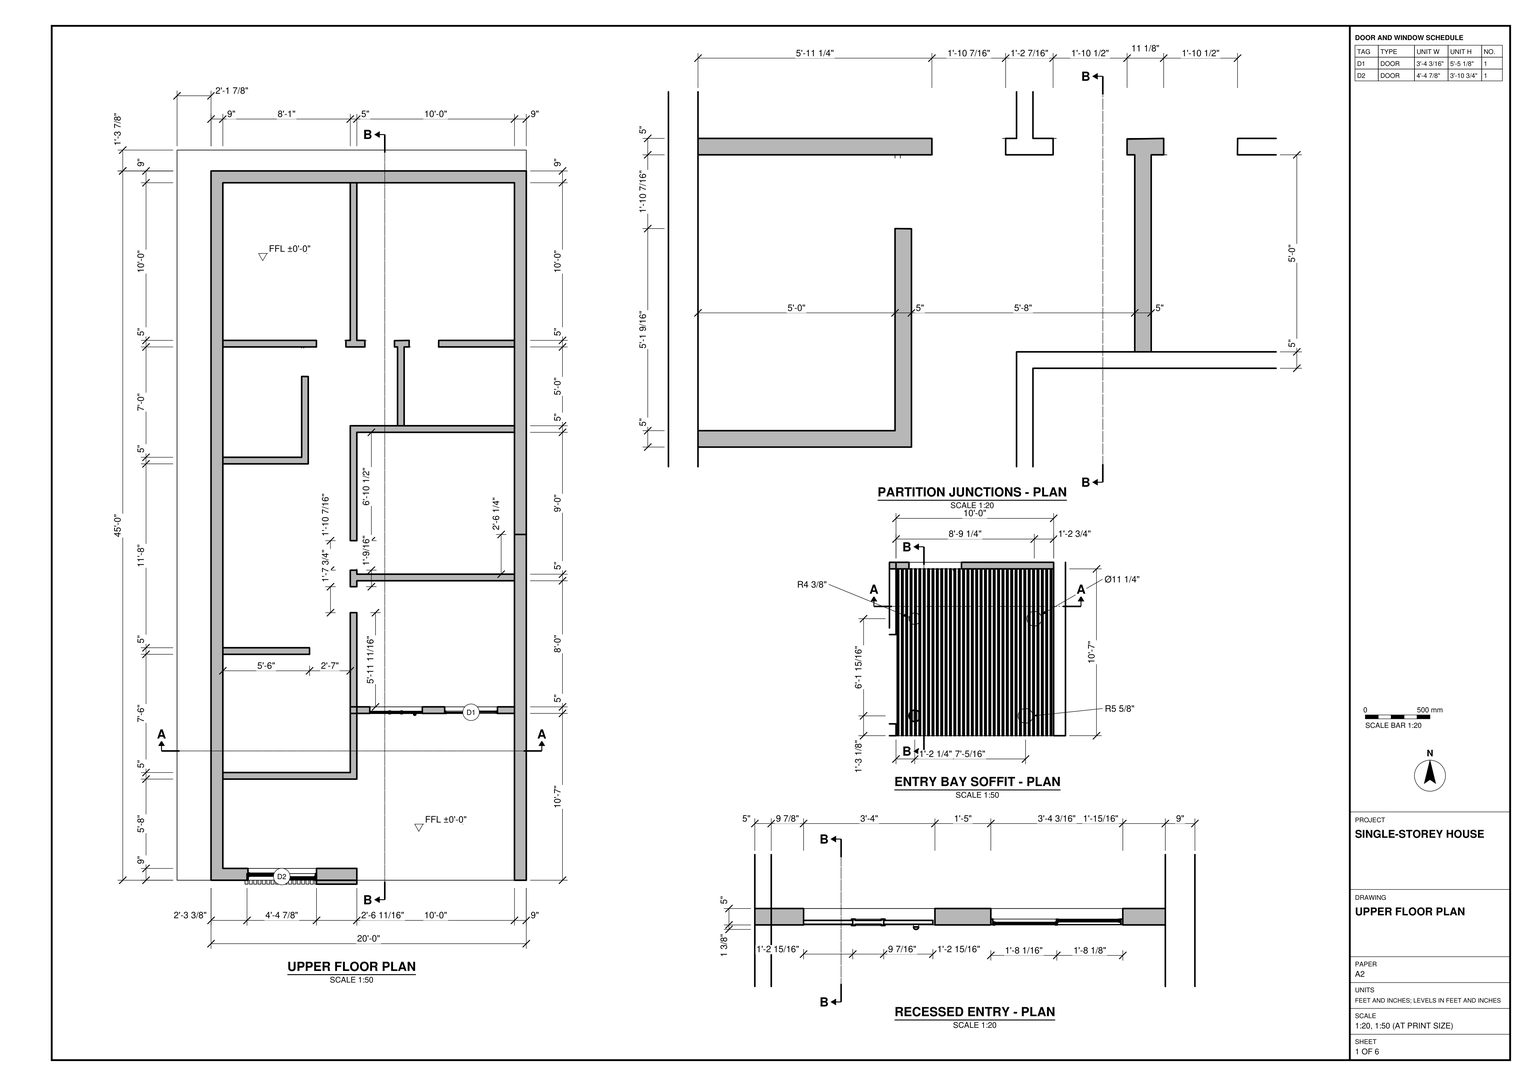
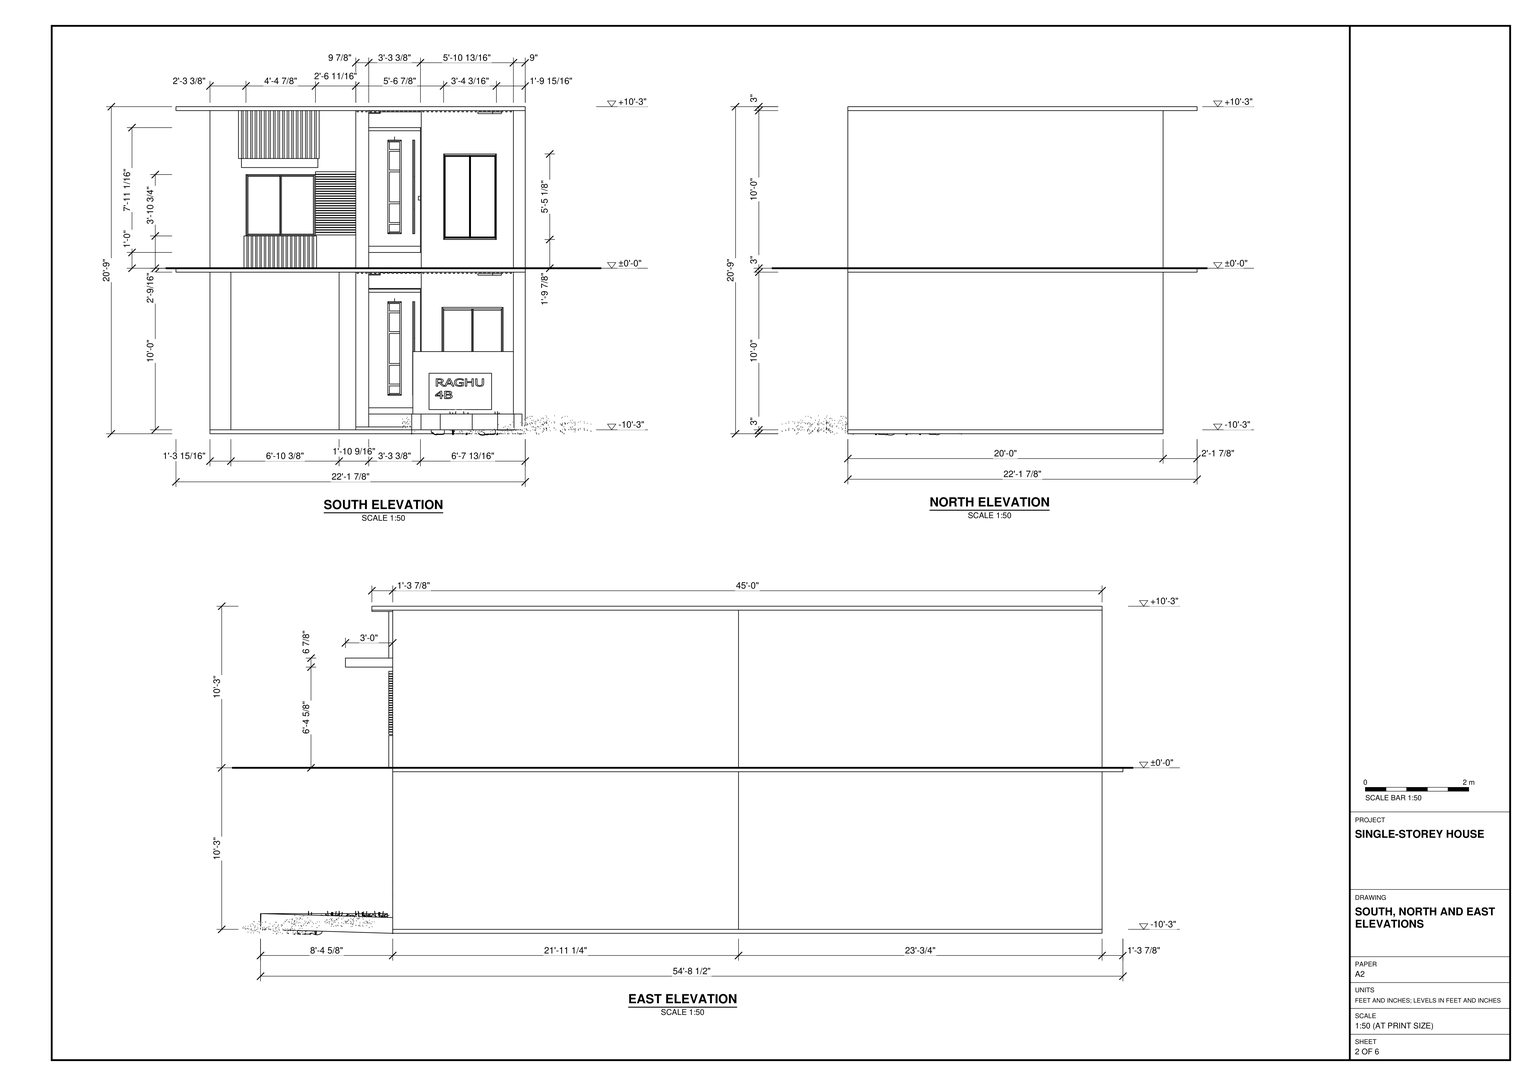
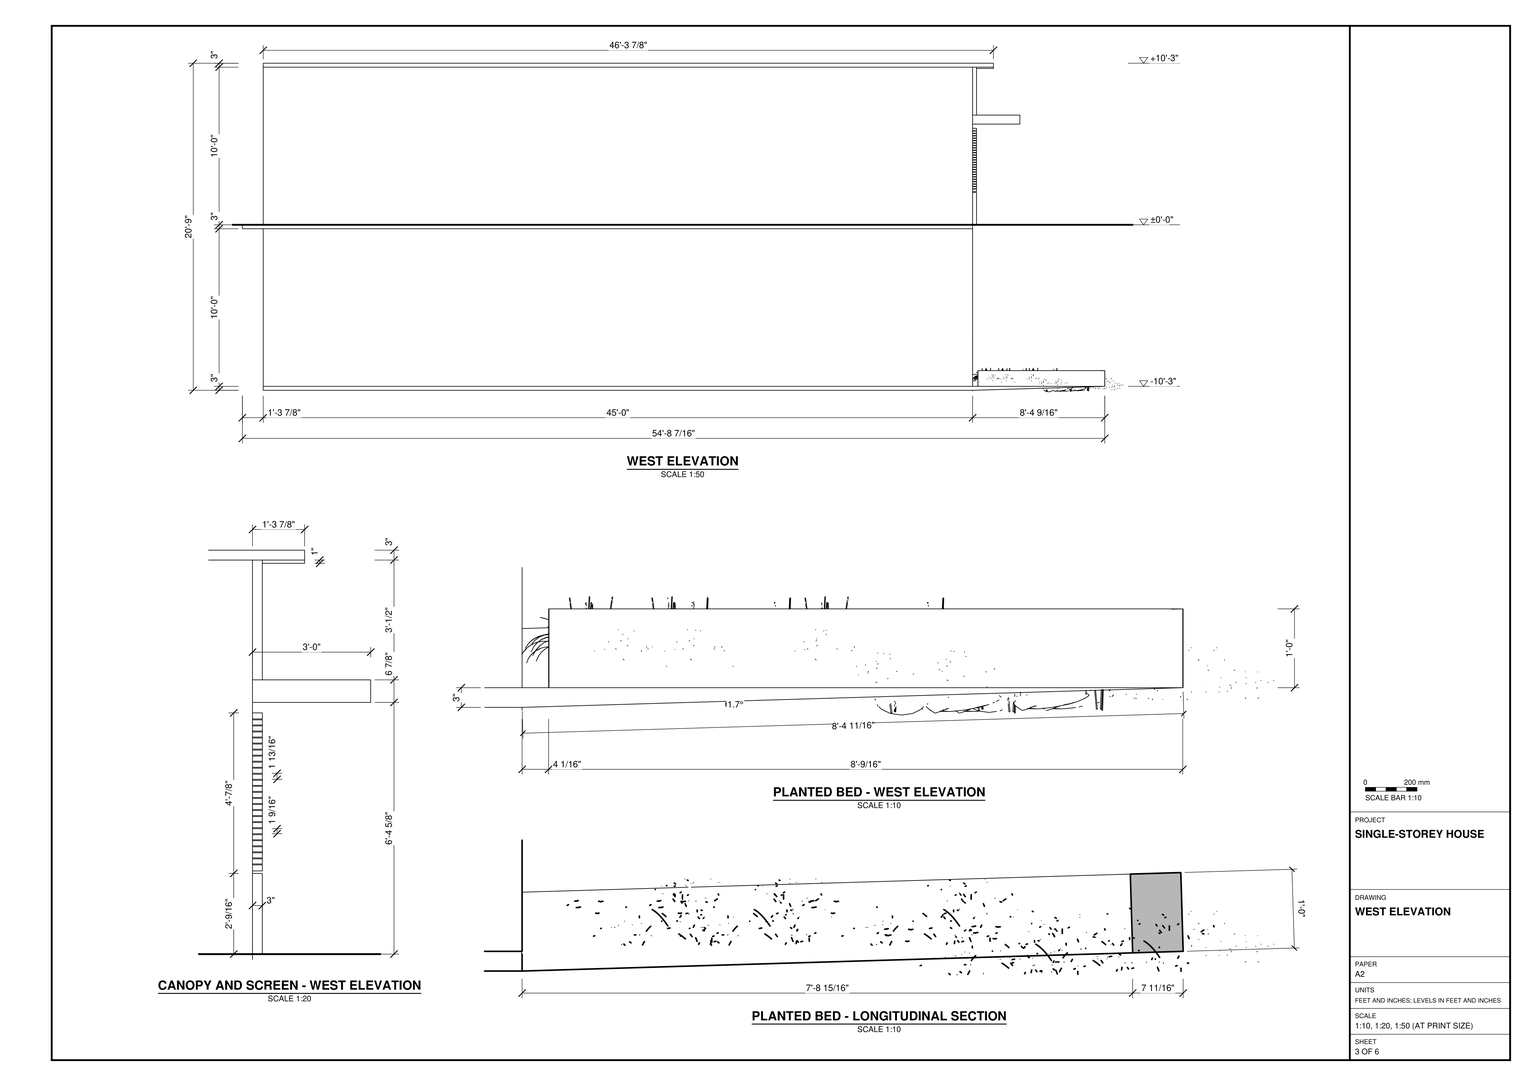
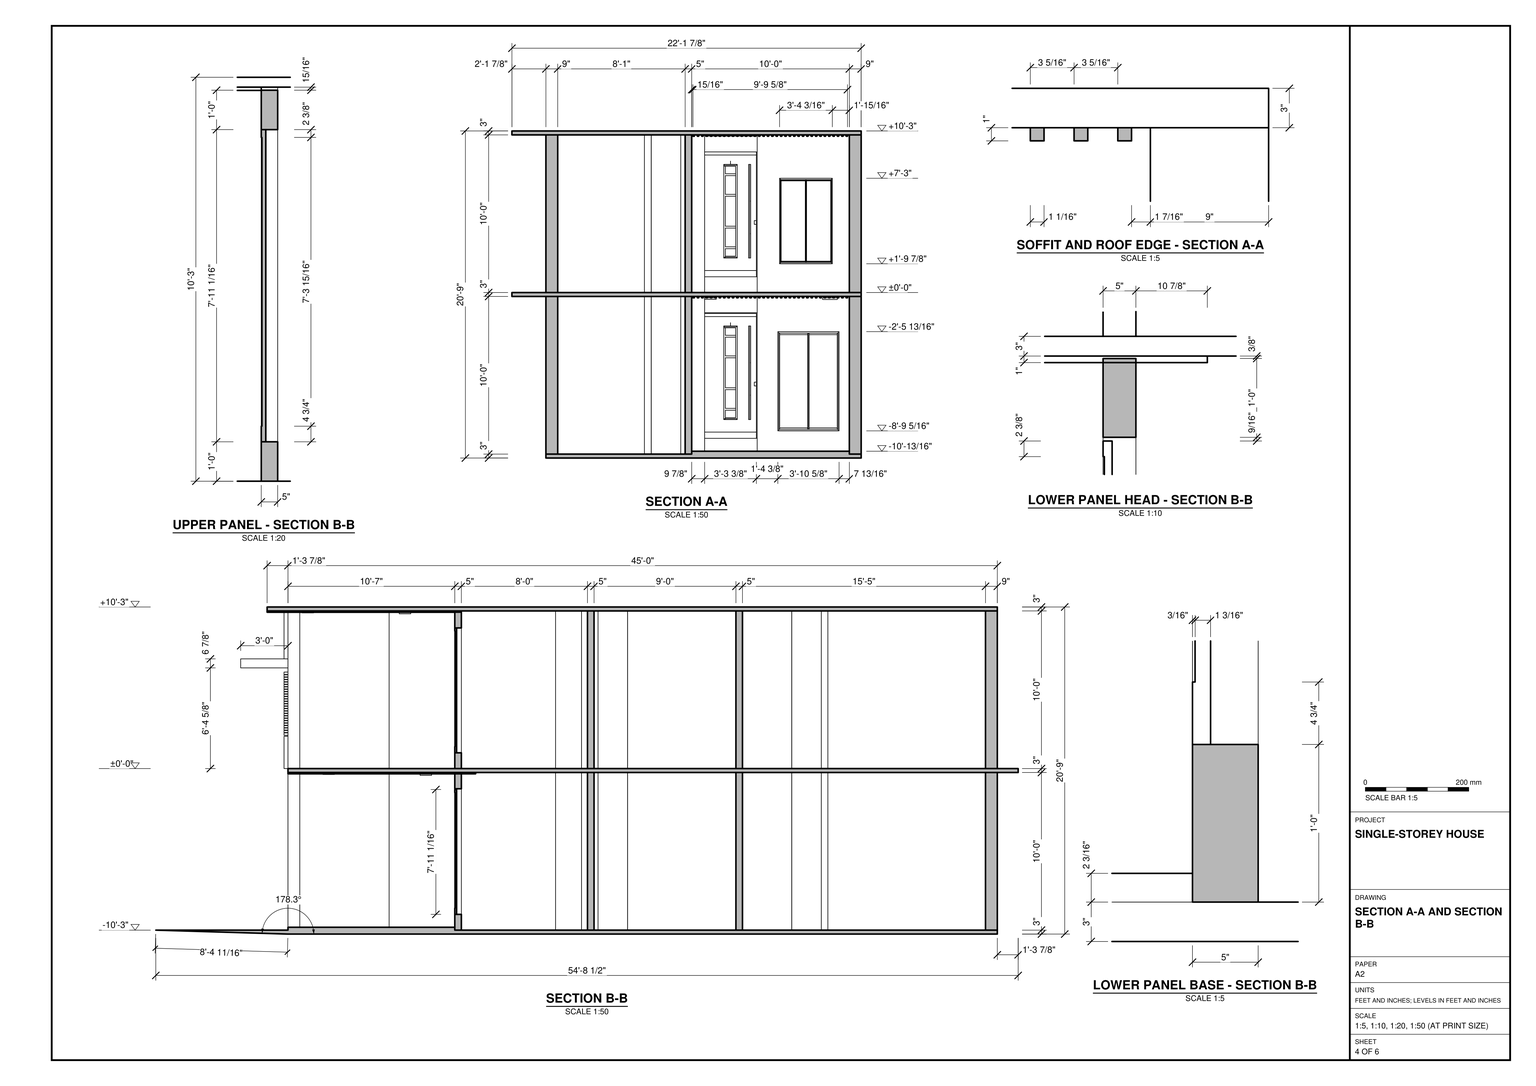
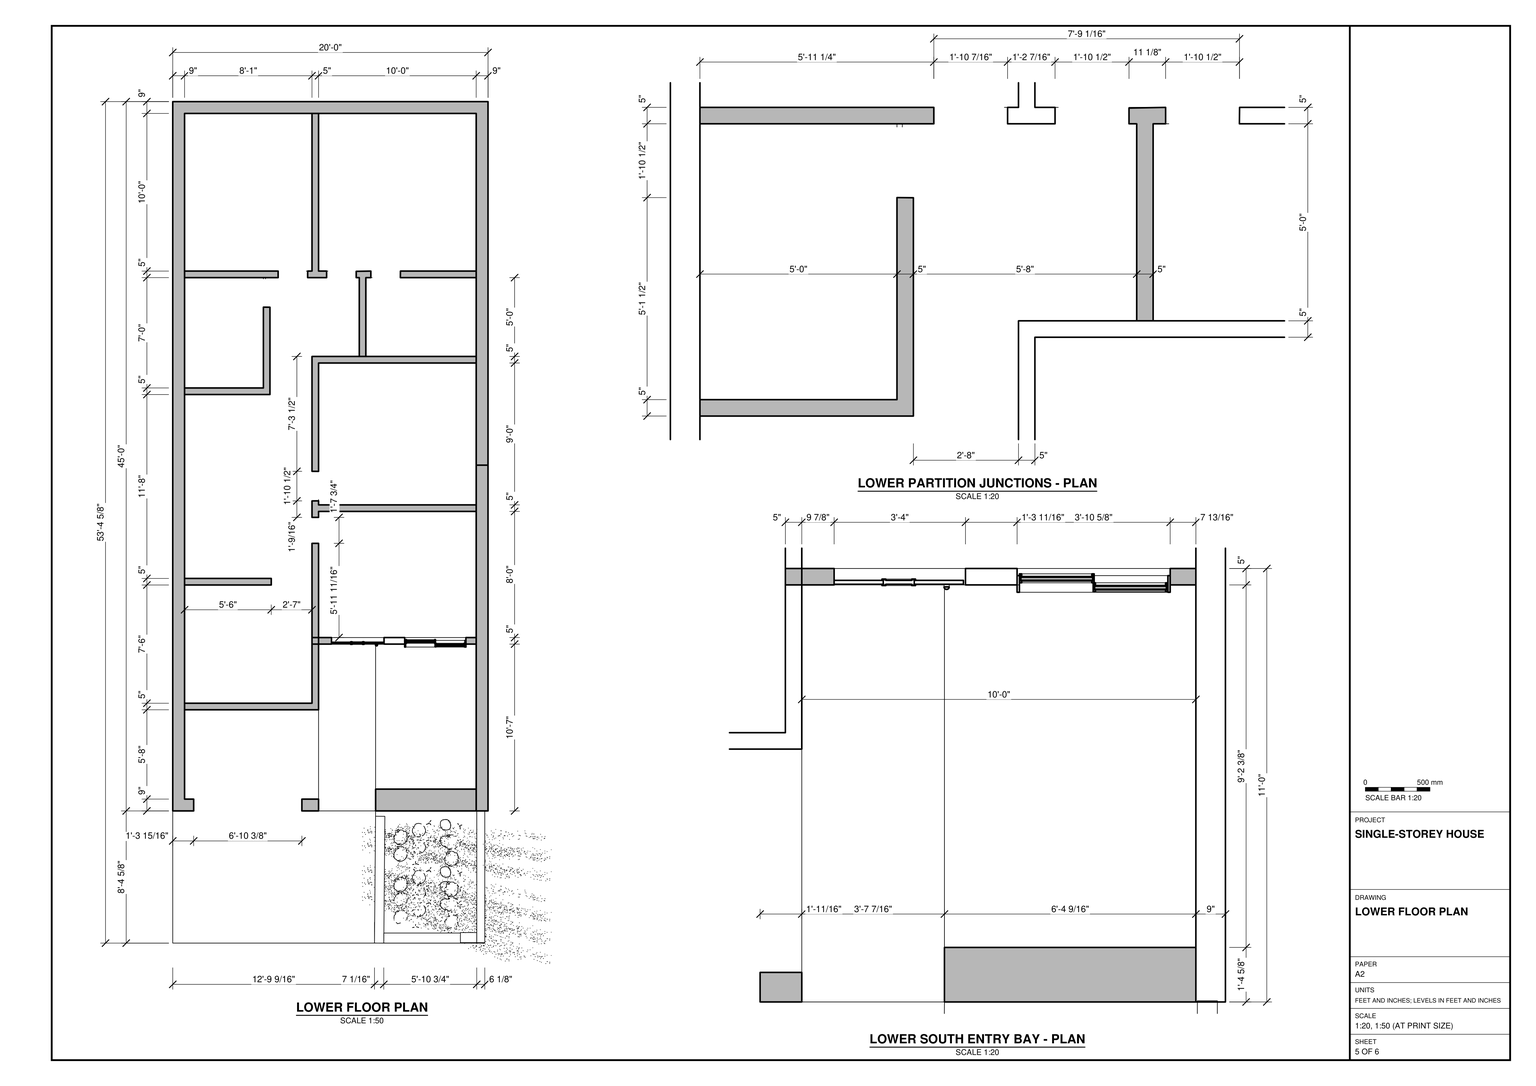
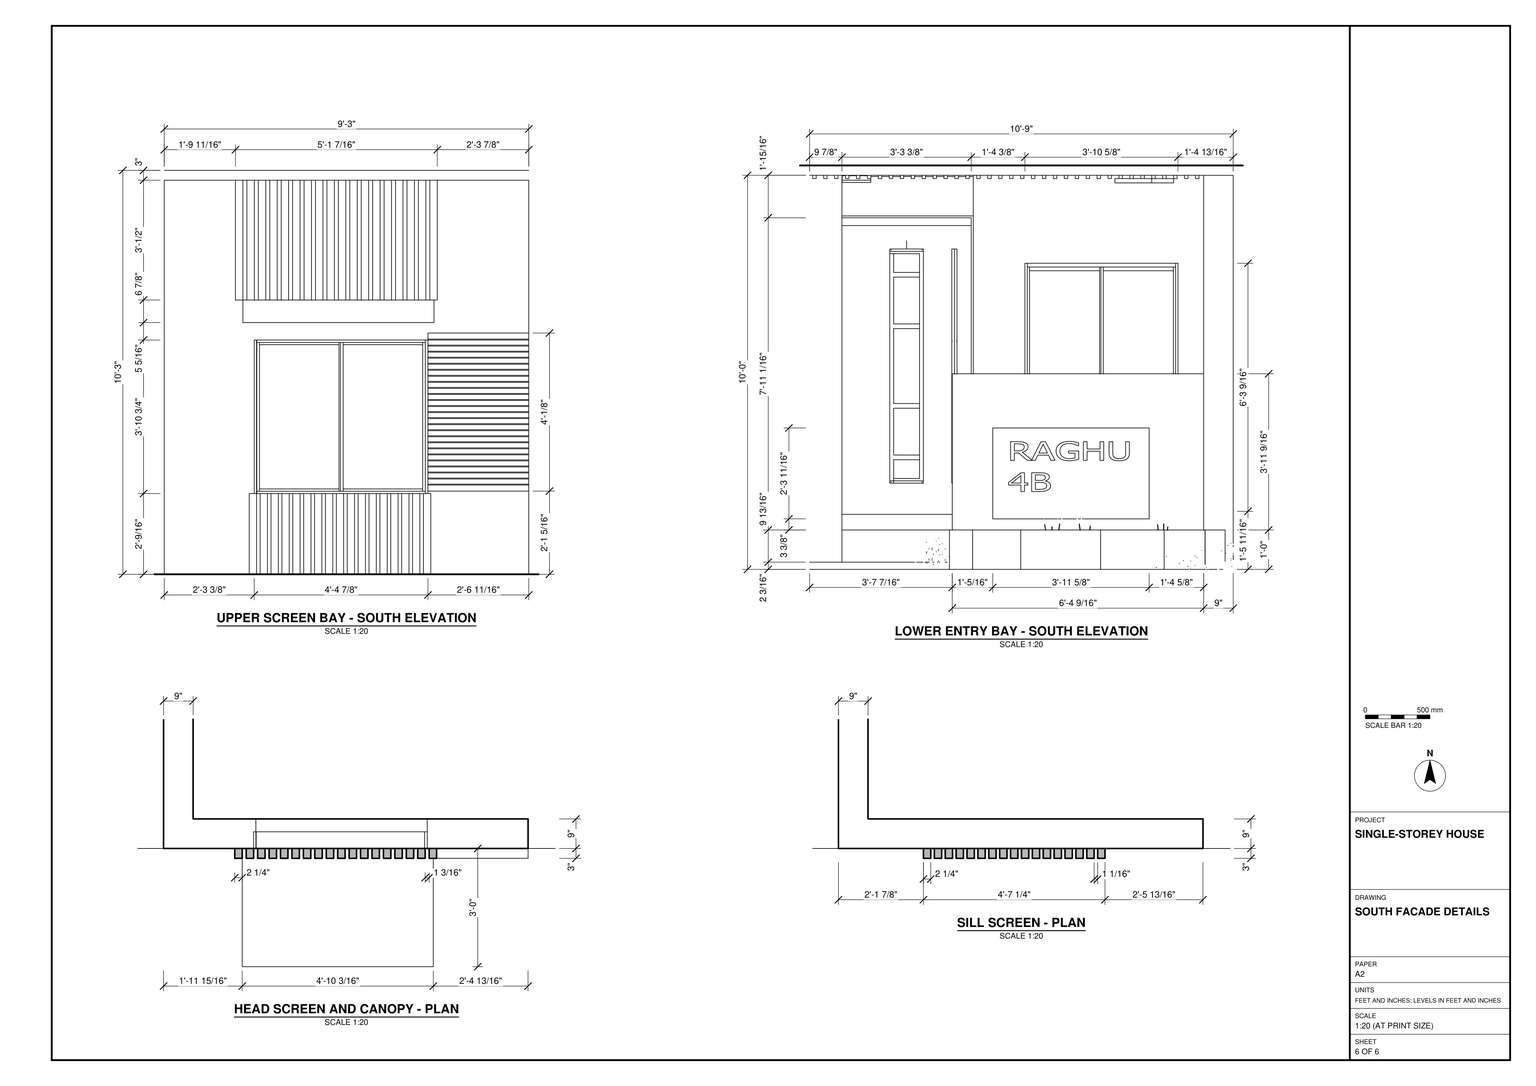
Build the house in SketchUp from task_files/diagram_01.pdf. Work in feet and inches. Use the finished floor of the partitioned plan as the ±0'-0" datum. The complete model, including projections and planting, measures 26'-4 5/16" across (x), 56'-2 5/16" front to back (y) and 20'-10 13/16" high (z).

Lay out the 20'-0" by 45'-0" house footprint with 9" exterior walls. Follow the plan and enlarged junction detail for the 5" partitions, including their short returns and the gaps between rooms. Use the elevations to build the enclosure below the datum floor as well as the walls above it. Match the thin slab edges and overhangs at the floor and flat roof; keep the side and rear walls plain as drawn.

On the south front, set the entrance back from the outer wall line. Model the framed openings, scheduled door units, slatted entry soffit, projecting canopy and screen. Use the south elevation to align the upper and lower entrance panels. Extend the low planted bed in front of the lower façade as shown in the west elevation and section. Decor and loose items, including plants, may be any suitable library components.

Keep walls, slabs, roof and each furniture or joinery piece shown in separate groups or components, and use components for repeated parts. Save one SketchUp model as output_files/house_with_its_recessed_entrance_and_planted_bed.skp.

# SketchUp Ruby script. Lengths in inches.
U = 1.inch
M = Sketchup.active_model
def pt(a) = Geom::Point3d.new(a.map { |v| v * U })
def face(e, loops, mat)
  f = e.add_face(loops[0].map { |a| pt(a) })
  loops[1..].each { |l| e.add_face(l.map { |a| pt(a) }).erase! }
  f.material = f.back_material = mat if mat
  f
end
# faces: each face lists its corners as indices into pts; further lists are holes
def faces(e, pts, list, mat = nil) = list.each { |f| face(e, (f[0].is_a?(Array) ? f : [f]).map { |l| l.map { |i| pts[i] } }, mat) }
# xy, xz, yz: faces in a plane at the given z, y or x. An outline is a flat list of corners, or four numbers for a rectangle; further outlines are holes
def ring(l) = l.size == 4 ? [[l[0], l[1]], [l[2], l[1]], [l[2], l[3]], [l[0], l[3]]] : l.each_slice(2).to_a
def flat(e, list, mat, &to3) = list.each { |f| face(e, (f[0].is_a?(Array) ? f : [f]).map { |l| ring(l).map { |u, v| to3.(u, v) } }, mat) }
def xy(e, z, list, mat = nil) = flat(e, list, mat) { |x, y| [x, y, z] }
def xz(e, y, list, mat = nil) = flat(e, list, mat) { |x, z| [x, y, z] }
def yz(e, x, list, mat = nil) = flat(e, list, mat) { |y, z| [x, y, z] }
def lines(e, pts, list) = list.each { |a, b| e.add_line(pt(pts[a]), pt(pts[b])) }
# prism: a flat outline (further loops are holes) pulled along v
def prism(e, loops, v, mat = nil)
  f = face(e, loops, mat); d = Geom::Vector3d.new(v.map { |x| x * U })
  f.pushpull(f.normal.samedirection?(d) ? d.length : -d.length)
end
def box(e, o, s, mat = nil) = prism(e, [[o, [o[0] + s[0], o[1], o[2]], [o[0] + s[0], o[1] + s[1], o[2]], [o[0], o[1] + s[1], o[2]]]], [0, 0, s[2]], mat)
def at(x, y, z, deg = 0) = Geom::Transformation.translation(pt([x, y, z])) * Geom::Transformation.rotation(ORIGIN, Z_AXIS, deg.degrees)
def axes(o, x, y, z) = Geom::Transformation.new([*x, 0, *y, 0, *z, 0, *pt(o).to_a, 1])
def part(name) = M.definitions.add(name)
# library, detail: a bought-in or finely detailed component or shape, given as its bounding box
def library(name, o, s) = part(name).tap { |d| box(d.entities, o, s) }
def detail(e, o, s) = box(e.add_group.entities, o, s)
def put(e, d, t, mat = nil) = e.add_instance(d, t).tap { |i| i.material = mat if mat }
def group(e, t, mat = nil) = e.add_group.tap { |g| g.transformation = t; g.material = mat if mat }.entities
root = M.entities
M.materials.add("Emissive\#1").color = [255, 185, 108]
M.materials.add("Glass_Tinted_Gray").color = [0, 0, 0]
M.materials["Glass_Tinted_Gray"].alpha = 0.125
M.materials.add("[0135_DarkGray]").color = [81, 81, 81]
M.materials.add("[Field Rectangle Tile]").color = [196, 189, 179]
M.materials.add("[Granite Dark Gray]").color = [69, 68, 68]
M.materials.add("[Marble Carrara Gold Floor Tile]").color = [225, 223, 217]
M.materials.add("[Mirror 02]").color = [229, 229, 229]
M.materials.add("[Terrazzo Light Blue]").color = [196, 214, 227]
M.materials.add("[Tile Navy]").color = [43, 47, 58]
M.materials.add("[Wood Bamboo]").color = [177, 105, 43]
M.materials.add("[Wood Veneer 01]").color = [120, 70, 37]
c1 = part("PENTEK_RP Fineline 50S_Sliding_DoorCase_E1")
box(c1.entities,[0,0,0],[1.51,3.66,99.27],"[0135_DarkGray]")
c2 = part("PENTEK_RP Fineline 50S_SlidingDooe_Case_E2")
box(c2.entities,[0,0,0],[96.25,3.66,1.51],"[0135_DarkGray]")
c3 = part("pentek_RP Fineline 50S_SlidingDoor_Case")
put(c3.entities,c1,at(97.76,0,0))
put(c3.entities,c2,at(1.51,0,0))
put(c3.entities,c1,at(0,0,0))
put(c3.entities,c2,at(1.51,0,97.76))
c4 = part("PENTEK_RP Fineline 50S_SlidingDoor_GlazingBead_2")
box(c4.entities,[0,0,0],[0.56,0.59,94.39],"[0135_DarkGray]")
c5 = part("PENTEK_RP Fineline 50S_SlidingDoor_Glass")
box(c5.entities,[0,0,0],[46.58,0.16,94.39],"Glass_Tinted_Gray")
c6 = part("PENTEK_RP Fineline 50S_SlidingDoor_GlazingBead")
box(c6.entities,[0,0,0],[45.47,0.59,0.56],"[0135_DarkGray]")
c7 = part("PENTEK_RP Fineline 50S_SlidingDoor_Leaf_E1")
xy(c7.entities,0,[[0,0,0.93,1.97],[0.93,1.57,1.49,1.97]],"[0135_DarkGray]")
xy(c7.entities,96.25,[[0,0,0.93,0,0.93,1.57,1.49,1.57,1.49,1.97,0,1.97]],"[0135_DarkGray]")
xz(c7.entities,0,[[0,0,0.93,96.25]],"[0135_DarkGray]")
xz(c7.entities,1.57,[[0.93,0,1.49,95.32],[0.93,95.32,1.49,96.25]],"[0135_DarkGray]")
xz(c7.entities,1.97,[[0,0,1.49,96.25]],"[0135_DarkGray]")
yz(c7.entities,0,[[0,0,1.97,96.25]],"[0135_DarkGray]")
yz(c7.entities,0.93,[[0,0,1.57,0.93],[0,0.93,1.57,95.32],[0,95.32,1.57,96.25]],"[0135_DarkGray]")
yz(c7.entities,1.49,[[1.57,0,1.97,95.32],[1.57,95.32,1.97,96.25]],"[0135_DarkGray]")
c8 = part("PENTEK_RP Fineline 50S_SlidingDoor_Leaf_E2")
xy(c8.entities,0,[[0,0,0,1.57,0.56,1.57,0.56,1.97,46.02,1.97,46.02,1.57,46.58,1.57,46.58,0]],"[0135_DarkGray]")
xy(c8.entities,0.93,[[0,0,46.58,1.57]],"[0135_DarkGray]")
xy(c8.entities,1.49,[[0.56,1.57,46.02,1.97]],"[0135_DarkGray]")
xz(c8.entities,0,[[0,0,46.58,0.93]],"[0135_DarkGray]")
xz(c8.entities,1.57,[[0,0,0.56,0.93],[46.02,0,46.58,0.93],[0.56,0.93,46.02,1.49]],"[0135_DarkGray]")
xz(c8.entities,1.97,[[0.56,0,46.02,1.49]],"[0135_DarkGray]")
yz(c8.entities,0,[[0,0,1.57,0.93]],"[0135_DarkGray]")
yz(c8.entities,0.56,[[1.57,0,1.97,0.93],[1.57,0.93,1.97,1.49]],"[0135_DarkGray]")
yz(c8.entities,46.02,[[1.57,0,1.97,0.93],[1.57,0.93,1.97,1.49]],"[0135_DarkGray]")
yz(c8.entities,46.58,[[0,0,1.57,0.93]],"[0135_DarkGray]")
c9 = part("PENTEK_RP Fineline S_SlidingDoor_Leaf1")
put(c9.entities,c4,at(0.93,0,0.93))
put(c9.entities,c4,at(46.96,0,0.93))
put(c9.entities,c5,at(1.49,1.42,0.93))
put(c9.entities,c6,at(1.49,0,0.93))
put(c9.entities,c5,at(1.49,0.59,0.93),"[Terrazzo Light Blue]")
put(c9.entities,c7,at(0,0,0))
put(c9.entities,c7,axes([48.44,0,0],[-1,0,0],[0,1,0],[0,0,1]))
put(c9.entities,c8,axes([0.93,0,96.25],[1,0,0],[0,1,0],[0,0,-1]))
put(c9.entities,c8,at(0.93,0,0))
put(c9.entities,c6,at(1.49,0,94.77))
c10 = part("PENTEK_RP Fineline 50S_SlidingDoor_Leaf2")
put(c10.entities,c5,at(1.49,1.42,0.93))
put(c10.entities,c6,at(1.49,0,94.77))
put(c10.entities,c4,at(46.96,0,0.93))
put(c10.entities,c5,at(1.49,0.59,0.93),"[Mirror 02]")
put(c10.entities,c4,at(0.93,0,0.93))
put(c10.entities,c7,at(0,0,0))
put(c10.entities,c7,axes([48.44,0,0],[-1,0,0],[0,1,0],[0,0,1]))
put(c10.entities,c6,at(1.49,0,0.93))
put(c10.entities,c8,axes([0.93,0,96.25],[1,0,0],[0,1,0],[0,0,-1]))
put(c10.entities,c8,at(0.93,0,0))
c11 = part("PENTEK - Slimmest Steel Sliding Door / Window\#1")
put(c11.entities,c3,at(0,-1.88,-0.09))
put(c11.entities,c9,at(1.51,-2.27,1.42))
put(c11.entities,c10,at(49.32,-0.3,1.42))
c12 = library("279",[-34.23,-17.84,-5],[65.55,41.78,17.48])
c13 = part("Group79\#1")
p = [[0,0,0],[0,0,-17.29],[-5.5625,0,-17.29],[36.2,-19.79,0],[-36.2,-19.79,0],[36.2,19.79,0],
  [36.2,0,0],[-36.2,19.79,0],[5.5625,0,-17.29],[-36.2,0,0],[0,0,-27.99]]
lines(c13.entities,p,[[0,1],[1,2],[3,4],[5,6],[7,5],[1,8],[9,0],[0,6],[8,10],[4,9],[6,3],[2,10],
  [9,7]])
c14 = part("Rectangle Light")
put(c14.entities,c13,at(0,0,0))
c15 = part("Group81\#1")
p = [[0,0,0],[0,0,-19.15],[-6.5,0,-19.15],[42.3,-19.6875,0],[-42.3,-19.6875,0],[42.3,19.6875,0],
  [42.3,0,0],[-42.3,19.6875,0],[6.5,0,-19.15],[-42.3,0,0],[0,0,-30.99]]
lines(c15.entities,p,[[0,1],[1,2],[3,4],[5,6],[7,5],[1,8],[9,0],[0,6],[8,10],[4,9],[6,3],[2,10],
  [9,7]])
c16 = part("Rectangle Light\#1")
put(c16.entities,c15,at(0,0,0))
c17 = part("Group83\#1")
p = [[0,0,0],[0,0,-18.71],[-5.84,0,-18.71],[38,-22.57,0],[-38,-22.57,0],[38,22.57,0],
  [38,0,0],[-38,22.57,0],[5.84,0,-18.71],[-38,0,0],[0,0,-30.28]]
lines(c17.entities,p,[[0,1],[1,2],[3,4],[5,6],[7,5],[1,8],[9,0],[0,6],[8,10],[4,9],[6,3],[2,10],
  [9,7]])
c18 = part("Rectangle Light\#2")
put(c18.entities,c17,at(0,0,0))
c19 = library("Entrance door",[0,-1.38,0],[39.37,3.16,78.74])
c20 = part("Group\#6")
prism(c20.entities,[[[11.15,65,0],[11.15,60,0],[7.35,60,0],[7.35,0,0],[2.35,0,0],[2.35,60,0],[0,60,0],[0,64.79,0]]],[0,0,120])
c21 = part("Group\#5")
prism(c21.entities,[[[0,0,0],[0.06,5,0],[57.73,5,0],[57.73,0,0]]],[0,0,120])
c22 = part("Group\#1")
box(c22.entities,[0,0,0],[5,5,120])
c23 = part("Group\#14")
prism(c23.entities,[[[71.23,0,0],[71.17,0,0],[0,0,0],[0,5,0],[71.23,5,0]]],[0,0,120])
c24 = part("Group\#2")
prism(c24.entities,[[[5,0,0],[0,0.04,0],[0,87.49,0],[36,87.49,0],[41,87.49,0],[125,87.49,0],[125,82.49,0],[5,82.49,0]]],[0,0,120])
c25 = part("Group\#4")
prism(c25.entities,[[[0,12.55,0],[5,12.58,0],[5,9.52,0],[125,9.52,0],[125,4.52,0],[5,4.52,0],[5,0,0],[0,0,0]]],[0,0,120])
c26 = part("Group\#3")
prism(c26.entities,[[[60,66.54,0],[65,66.48,0],[65,0,0],[0,0,0],[0,5,0],[60,5,0]]],[0,0,120])
c27 = part("Group\#13")
box(c27.entities,[0,0,0],[5,71.71,120])
c28 = part("Group\#9")
box(c28.entities,[0,0,0],[65.99,5,120])
c29 = part("Group\#10")
box(c29.entities,[0,0,0],[9.85,5,120])
c30 = part("Group\#21")
box(c30.entities,[0,0,0],[40,5,12])
c31 = part("Group\#24")
box(c31.entities,[0,0,0],[2.27,3,36.48])
c32 = part("Group\#25")
box(c32.entities,[0,0,0],[2.23,3,24.58])
c33 = part("Group\#26")
box(c33.entities,[0,0,0],[30.7,3,2.13])
c34 = part("Group\#29")
box(c34.entities,[0,0,0],[1.05,142.875,1])
c35 = library("Group\#31",[0,0,0],[100.96,85.18,2.1875])
c36 = part("Group\#32")
g1 = group(c36.entities,at(0,0,1.3125))
g2 = group(g1,at(25.875,15.875,4))
box(g2,[-25.875,-15.875,-3],[265.875,555.875,3])
put(g1,c34,at(141.16,0,0))
g3 = group(g1,at(161.14,0,0))
box(g3,[0,0,0],[1.05,142.875,1])
put(g1,c34,at(184.46,0,0))
put(g1,c34,at(167.81,0,0))
put(g1,c34,at(197.78,0,0))
put(g1,c34,at(211.1,0,0))
put(g1,c34,at(221.09,0,0))
put(g1,c34,at(231.08,0,0))
put(g1,c34,at(227.75,0,0))
put(g1,c34,at(171.14,0,0))
put(g1,c34,at(204.44,0,0))
put(g1,c34,at(234.41,0,0))
put(g1,c34,at(157.81,0,0))
put(g1,c34,at(214.43,0,0))
put(g1,c34,at(164.48,0,0))
put(g1,c34,at(181.13,0,0))
put(g1,c34,at(201.11,0,0))
put(g1,c34,at(217.76,0,0))
put(g1,c34,at(241.07,0,0))
put(g1,c34,at(144.49,0,0))
put(g1,c34,at(194.45,0,0))
put(g1,c34,at(244.4,0,0))
put(g1,c34,at(147.82,0,0))
put(g1,c34,at(151.15,0,0))
put(g1,c34,at(207.77,0,0))
put(g1,c34,at(224.42,0,0))
put(g1,c34,at(237.74,0,0))
put(g1,c34,at(154.48,0,0))
put(g1,c34,at(174.47,0,0))
put(g1,c34,at(177.8,0,0))
put(g1,c34,at(187.79,0,0))
put(g1,c34,at(191.12,0,0))
put(g1,c34,at(251.06,0,0))
put(g1,c34,at(247.73,0,0))
put(g1,c34,at(254.39,0,0))
put(g1,c34,at(137.83,0,0))
put(c36.entities,c35,at(146.78,25.38,0))
xy(root,-3,[[25.875,100.65,265.875,640.65]])
xy(root,0,[[186.53,0,186.53,0.02,183.9,0.02],[186.53,0,244.84,0.02],[244.84,0,257.29,0.02],[179.47,0.02,179.47,0.06,183.9,0.02],[183.9,0.02,186.53,0.02,186.53,7.6875,186.59,7.6875,187.34,96.55,180.28,96.61,179.47,0.06],
  [186.53,0.02,186.59,7.6875,186.53,7.6875],[186.53,0.02,244.84,0.02,244.84,7.6875,186.59,7.6875],[180.3125,100.65,256.875,117.25],[128.56,506.65,128.56,511.65,131.875,511.65,131.875,631.65,136.875,631.65,136.875,511.65,143.01,511.65,143.01,506.65]])
xy(root,0,[[[25.875,0.02,25.875,640.65,265.875,640.65,265.875,100.65,256.875,100.65,256.875,227.65,136.875,227.65,136.875,100.65,180.3125,100.65,180.28,96.61,179.47,0.06,179.47,0.02],[128.56,506.65,143.01,506.65,143.01,511.65,136.875,511.65,136.875,631.65,131.875,631.65,131.875,511.65,128.56,511.65]]],"[Tile Navy]")
xy(root,2.1875,[[180.3125,117.25,256.875,227.65]],"[Marble Carrara Gold Floor Tile]")
xy(root,12,[[186.53,0,186.53,7.6875,186.59,7.6875,187.34,96.55,180.28,96.61,179.47,0.06],[186.53,0,244.84,0,244.84,7.6875,186.59,7.6875]])
xy(root,59.5625,[[180.3125,100.65,256.875,117.25]])
xy(root,120,[[128.56,506.65,143.01,506.65,143.01,511.65,136.875,511.65,136.875,631.65,131.875,631.65,131.875,511.65,128.56,511.65]])
xy(root,242,[[235.46,110.16,236.91,110.35,238.27,110.91,239.43,111.8,240.32,112.96,240.88,114.32,241.07,115.77,240.88,117.22,240.32,118.58,239.43,119.74,238.27,120.63,236.91,121.2,235.46,121.39,234,121.2,232.65,120.63,231.49,119.74,230.6,118.58,230.03,117.22,229.84,115.77,230.03,114.32,230.6,112.96,231.49,111.8,232.65,110.91,234,110.35],[242.12,184.1,243.57,184.29,244.93,184.86,246.09,185.75,246.98,186.91,247.54,188.27,247.73,189.72,247.54,191.17,246.98,192.53,246.09,193.6875,244.93,194.58,243.57,195.14,242.12,195.33,240.67,195.14,239.3125,194.58,238.15,193.6875,237.26,192.53,236.69,191.17,236.5,189.72,236.69,188.27,237.26,186.91,238.15,185.75,239.3125,184.86,240.67,184.29],[151.15,185.34,152.29,185.49,153.34,185.93,154.25,186.625,154.94,187.53,155.38,188.59,155.53,189.72,155.38,190.85,154.94,191.91,154.25,192.8125,153.34,193.51,152.29,193.95,151.15,194.09,150.02,193.95,148.97,193.51,148.06,192.8125,147.36,191.91,146.93,190.85,146.78,189.72,146.93,188.59,147.36,187.53,148.06,186.625,148.97,185.93,150.02,185.49]],"Emissive\#1")
xz(root,0,[[186.53,0,201.17,12],[201.17,0,225.51,12],[225.51,0,244.84,12]])
xz(root,7.6875,[[186.53,0,186.59,12],[186.59,0,244.84,12]])
xz(root,100.65,[[179.47,-3,265.875,-3,265.875,0],[136.875,0,180.3125,2.1875]])
xz(root,117.25,[[180.3125,0,256.875,2.1875],[180.3125,2.1875,256.875,59.5625]])
xz(root,227.65,[[136.875,0,256.875,2.1875]])
xz(root,506.65,[[128.56,0,143.01,120]])
xz(root,511.65,[[128.56,0,131.875,120],[136.875,0,143.01,120]])
xz(root,631.65,[[131.875,0,136.875,120]])
xz(root,640.65,[[25.875,-3,265.875,0]])
yz(root,25.875,[[100.65,-3,0.02,0,640.65,0,640.65,-3]])
yz(root,128.56,[[506.65,0,511.65,120]])
yz(root,131.875,[[511.65,0,631.65,120]])
yz(root,136.875,[[100.65,0,227.65,2.1875],[511.65,0,631.65,120]])
yz(root,143.01,[[506.65,0,511.65,120]])
yz(root,180.3125,[[100.65,0,117.25,2.1875],[100.65,2.1875,117.25,59.5625]])
yz(root,186.53,[[0,0,7.6875,12]])
yz(root,244.84,[[7.6875,-0.23,0.02,0,0,0,0.36,11.99,7.6875,11.78,8.04,11.77],[0,0,7.6875,12]])
yz(root,256.875,[[100.65,0,117.25,59.5625],[117.25,0,227.65,2.1875]])
yz(root,257.29,[[7.6875,-0.23,8.04,11.77,0.36,11.99,0,0,0.02,0]])
yz(root,257.33,[[100.65,-3,0.02,0,0,0,0.36,11.99,101,8.99]])
yz(root,263.41,[[100.65,-3,101,8.99,0.36,11.99,0,0]])
yz(root,265.875,[[100.65,-3,640.65,0]])
p = [[179.47,100.65,-3],[179.47,0.02,0],[25.875,0.02,0],[25.875,100.65,-3],[257.33,100.65,-3],[257.33,0.02,0],
  [257.29,0.02,0],[257.29,7.6875,-0.23],[244.84,7.6875,-0.23],[244.84,0.02,0],[186.53,0.02,0],[183.9,0.02,0],
  [257.33,0,0],[263.41,100.65,-3],[263.41,0,0],[257.33,101,8.99],[263.41,101,8.99],[244.84,8.04,11.77],
  [257.29,8.04,11.77],[179.47,0.06,0],[186.53,0,0],[186.53,0,12],[179.47,0.06,12],[186.59,7.6875,12],
  [186.59,7.6875,0],[244.84,0,0],[257.29,0,0],[257.29,0.36,11.99],[244.84,0.36,11.99],[263.41,0.36,11.99],
  [257.33,0.36,11.99],[180.28,96.61,0],[180.28,96.61,12],[187.34,96.55,0],[187.34,96.55,12],[244.84,7.6875,11.78],
  [176.68,506.65,0],[177.67,506.65,0],[143.01,511.65,0],[144,511.65,0],[96.5,505.66,0],[96.5,506.65,0],
  [136.875,337.69,0],[136.875,336.71,0],[127.57,511.65,0],[128.56,511.65,0],[165.47,511.65,0],[176.68,511.65,0],
  [94.875,505.66,0],[94.875,506.65,0],[179.47,100.65,-3.4375]]
faces(root,p,[[0,1,2,3],[0,4,5,6,7,8,9,10,11,1],[12,5,4,13,14],[13,4,15,16],[7,6,9,8],[7,8,17,18],[19,11,20,21,22],[10,20,21,23,24],
  [25,26,27,28],[12,14,29,30],[31,19,22,32],[24,33,34,23],[33,31,32,34],[15,30,29,16],[35,28,27,18,17]])
lines(root,p,[[36,37],[38,39],[40,41],[42,43],[44,45],[46,47],[48,49],[0,50]])
detail(root,[192.65,100.65,15.375],[47.63,2,27.6875])
put(root,c11,axes([203.74,228.65,144.94],[0.40482,0,0],[0,0.44,0],[0,0,0.65593]))
put(root,c11,axes([53.28,103.12,147.625],[0.53284,0,0],[0,-1.38599,0],[0,0,0.47093]))
put(root,c3,axes([202.44,230.47,17.68],[0.46959,0,0],[0,-1.38599,0],[0,0,0.76088]))
put(root,c9,axes([203.15,231.02,18.83],[0.46959,0,0],[0,-1.38599,0],[0,0,0.76088]))
put(root,c10,axes([225.6,228.29,18.83],[0.46959,0,0],[0,-1.38599,0],[0,0,0.76088]))
put(root,c12,at(226,68.16,3.33))
put(root,c12,at(226,44.85,3.33))
put(root,c12,at(226,33.53,-0.94))
put(root,c12,at(226,20.22,-0.54))
put(root,c12,at(226,80.73,3.33))
put(root,c14,at(188.17,294.38,119.99))
put(root,c16,at(190.61,284.2,242.99))
put(root,c18,axes([72.87,144.89,242.99],[-1,0,0],[0,1,0],[0,0,1]))
put(root,c19,axes([146.72,227.65,135],[1,0,0],[0,1,0],[0,0,1.20729]))
put(root,c19,axes([146.72,227.65,12],[1,0,0],[0,1,0],[0,0,1.20729]))
g4 = group(root,at(25.875,100.65,123))
prism(g4,[[[102.69,406,0],[102.69,411,0],[106,411,0],[106,531,0],[111,531,0],[111,411,0],[117.13,411,0],[117.13,406,0]]],[0,0,120])
p = [[150.81,406,0],[151.79,406,0],[117.13,411,0],[118.12,411,0],[70.62,405.01,0],[70.62,406,0],
  [111,237.05,0],[111,236.06,0],[101.7,411,0],[102.69,411,0],[139.59,411,0],[150.81,411,0],
  [69,405.01,0],[69,406,0]]
lines(g4,p,[[0,1],[2,3],[4,5],[6,7],[8,9],[10,11],[12,13]])
g5 = group(g4,at(9,77,0))
prism(g5,[[[102,0,0],[0,0,0],[0,5,0],[97,5,0],[97,50,0],[102,50,0]]],[0,0,120])
g6 = group(g4,at(231,0,0))
prism(g6,[[[0,127,0],[0,132,0],[0,228,0],[0,233,0],[0,263.24,0],[9,263.24,0],[9,0,0],[0,0,0]]],[0,0,120])
g7 = group(g4,at(160.85,127,0))
prism(g7,[[[0,0,0],[70.15,0,0],[70.15,0,120],[0,0,120]],[[57.2,0,21.97],[17.02,0,21.97],[17.02,0,87],[57.2,0,87]]],[0,5,0])
g8 = group(g4,at(0,0,0))
xy(g8,0,[[0,0,0,540,240,540,240,263.24,231,263.24,231,531,9,531,9,9,111,9,111,0]])
xy(g8,24.58,[[28.11,0,80.3,9]])
xy(g8,71.33,[[28.11,0,80.3,9]])
xy(g8,120,[[0,0,111,0,111,9,9,9,9,531,231,531,231,263.24,240,263.24,240,540,0,540]])
xz(g8,0,[[[0,0,111,120],[28.11,24.58,80.3,71.33]]])
xz(g8,9,[[[9,0,111,120],[28.11,24.58,80.3,71.33]]])
xz(g8,263.24,[[231,0,240,120]])
xz(g8,531,[[9,0,106,120],[106,0,111,120],[111,0,231,120]])
xz(g8,540,[[0,0,240,120]])
yz(g8,0,[[0,0,540,120]])
yz(g8,9,[[9,0,77,120],[77,0,82,120],[82,0,172,120],[172,0,177,120],[177,0,531,120]])
yz(g8,28.11,[[0,24.58,9,71.33]])
yz(g8,80.3,[[0,24.58,9,71.33]])
yz(g8,111,[[0,0,9,120]])
yz(g8,231,[[263.24,0,341,120],[341,0,346,120],[346,0,406,120],[406,0,411,120],[411,0,531,120]])
yz(g8,240,[[263.24,0,540,120]])
put(g4,c20,at(139.65,346,0))
put(g4,c21,at(173.27,406,0))
put(g4,c22,at(106,127,0))
put(g4,c23,at(9,406,0))
put(g4,c24,at(106,258.51,0))
put(g4,c25,at(106,223.48,0))
put(g4,c26,at(9,317,0))
put(g4,c27,at(106,132,0))
put(g4,c28,at(9,172,0))
put(g4,c29,at(111,127,0))
put(root,c30,at(146.72,227.65,0))
put(root,c30,at(146.72,227.65,107.625))
put(root,c30,at(146.72,227.65,123))
put(root,c30,at(146.72,227.65,230.0625))
g9 = group(root,at(49.83,64.65,199.64),"[Wood Veneer 01]")
detail(g9,[0,0,0],[58.1875,36,6.875])
g10 = group(root,at(47.5625,97.65,206.52),"[Wood Bamboo]")
box(g10,[0,0,0],[2.27,3,36.48])
put(root,c31,at(51.04,97.65,206.52),"[Wood Bamboo]")
put(root,c31,at(54.53,97.65,206.52),"[Wood Bamboo]")
put(root,c31,at(58.01,97.65,206.52),"[Wood Bamboo]")
put(root,c31,at(61.49,97.65,206.52),"[Wood Veneer 01]")
put(root,c31,at(64.97,97.65,206.52),"[Wood Bamboo]")
put(root,c31,at(68.45,97.65,206.52),"[Wood Bamboo]")
put(root,c31,at(71.9375,97.65,206.52),"[Wood Bamboo]")
put(root,c31,at(75.42,97.65,206.52),"[Wood Veneer 01]")
put(root,c31,at(78.9,97.65,206.52),"[Wood Bamboo]")
put(root,c31,at(82.38,97.65,206.52),"[Wood Bamboo]")
put(root,c31,at(85.86,97.65,206.52),"[Wood Bamboo]")
put(root,c31,at(89.34,97.65,206.52),"[Wood Bamboo]")
put(root,c31,at(92.83,97.65,206.52),"[Wood Bamboo]")
put(root,c31,at(96.31,97.65,206.52),"[Wood Bamboo]")
put(root,c31,at(99.79,97.65,206.52),"[Wood Bamboo]")
put(root,c31,at(103.27,97.65,206.52),"[Wood Bamboo]")
put(root,c31,at(106.75,97.65,206.52),"[Wood Bamboo]")
put(root,c32,at(51.76,97.65,123),"[Wood Bamboo]")
put(root,c32,at(55.07,97.65,123),"[Wood Bamboo]")
put(root,c32,at(58.39,97.65,123),"[Wood Bamboo]")
put(root,c32,at(61.7,97.65,123),"[Wood Bamboo]")
put(root,c32,at(65.02,97.65,123),"[Wood Bamboo]")
put(root,c32,at(68.33,97.65,123),"[Wood Bamboo]")
put(root,c32,at(71.65,97.65,123),"[Wood Bamboo]")
put(root,c32,at(74.97,97.65,123),"[Wood Bamboo]")
put(root,c32,at(78.28,97.65,123),"[Wood Bamboo]")
put(root,c32,at(81.6,97.65,123),"[Wood Bamboo]")
put(root,c32,at(84.91,97.65,123),"[Wood Bamboo]")
put(root,c32,at(88.23,97.65,123),"[Wood Bamboo]")
put(root,c32,at(91.54,97.65,123),"[Wood Bamboo]")
put(root,c32,at(94.86,97.65,123),"[Wood Bamboo]")
put(root,c32,at(98.17,97.65,123),"[Wood Bamboo]")
put(root,c32,at(101.49,97.65,123),"[Wood Bamboo]")
put(root,c32,at(104.81,97.65,123),"[Wood Bamboo]")
put(root,c33,at(106.17,97.65,194.33),"[Wood Bamboo]")
put(root,c33,at(106.17,97.65,192.49),"[Wood Bamboo]")
put(root,c33,at(106.17,97.65,190.65),"[Wood Bamboo]")
put(root,c33,at(106.17,97.65,188.81),"[Wood Bamboo]")
put(root,c33,at(106.17,97.65,186.97),"[Wood Bamboo]")
put(root,c33,at(106.17,97.65,185.13),"[Wood Bamboo]")
put(root,c33,at(106.17,97.65,183.29),"[Wood Bamboo]")
put(root,c33,at(106.17,97.65,181.45),"[Wood Bamboo]")
put(root,c33,at(106.17,97.65,179.61),"[Wood Bamboo]")
put(root,c33,at(106.17,97.65,177.77),"[Wood Bamboo]")
put(root,c33,at(106.17,97.65,175.93),"[Wood Bamboo]")
put(root,c33,at(106.17,97.65,174.09),"[Wood Bamboo]")
put(root,c33,at(106.17,97.65,172.25),"[Wood Bamboo]")
put(root,c33,at(106.17,97.65,170.41),"[Wood Bamboo]")
put(root,c33,at(106.17,97.65,168.57),"[Wood Bamboo]")
put(root,c33,at(106.17,97.65,166.73),"[Wood Bamboo]")
put(root,c33,at(106.17,97.65,164.89),"[Wood Bamboo]")
put(root,c33,at(106.17,97.65,163.05),"[Wood Bamboo]")
put(root,c33,at(106.17,97.65,161.21),"[Wood Bamboo]")
put(root,c33,at(106.17,97.65,159.37),"[Wood Bamboo]")
put(root,c33,at(106.17,97.65,157.53),"[Wood Bamboo]")
put(root,c33,at(106.17,97.65,155.69),"[Wood Bamboo]")
put(root,c33,at(106.17,97.65,153.85),"[Wood Bamboo]")
put(root,c33,at(106.17,97.65,152.01),"[Wood Bamboo]")
put(root,c33,at(106.17,97.65,150.17),"[Wood Bamboo]")
put(root,c33,at(106.17,97.65,148.33),"[Wood Bamboo]")
put(root,c36,at(0,84.77,240.6875),"[Wood Bamboo]")
put(root,c36,at(0,100.65,117.6875),"[Wood Bamboo]")
g11 = group(root,at(180.3125,100.65,0))
xz(g11,0,[[[0,0,76.5625,59.5625],[12.34,15.375,59.96,43.0625]]])
g12 = group(root,at(34.875,177.65,0))
prism(g12,[[[102,0,0],[0,0,0],[0,5,0],[97,5,0],[97,50,0],[102,50,0]]],[0,0,120])
g13 = group(root,at(256.875,100.65,0))
prism(g13,[[[0,127,0],[0,132,0],[0,228,0],[0,233,0],[0,263.24,0],[9,263.24,0],[9,0,0],[0,0,0]]],[0,0,120])
g14 = group(root,at(186.72,227.65,0))
prism(g14,[[[0,0,0],[70.15,0,0],[70.15,0,120],[0,0,120]],[[62.34,0,17.77],[15.71,0,17.77],[15.71,0,93.21],[62.34,0,93.21]]],[0,5,0])
g15 = group(root,at(25.875,100.65,0))
prism(g15,[[[9,9,0],[15.93,9,0],[15.93,0,0],[0,0,0],[0,540,0],[240,540,0],[240,263.24,0],[231,263.24,0],[231,341,0],[231,346,0],[231,406,0],[231,411,0],[231,531,0],[111,531,0],[106,531,0],[9,531,0],[9,177,0],[9,172,0],[9,82,0],[9,77,0]]],[0,0,120])
box(g15,[98.31,0,0],[12.69,9,120])
p = [[98.31,9,120],[15.93,9,120]]
lines(g15,p,[[0,1]])
put(root,c20,at(165.53,446.65,0))
put(root,c21,at(199.14,506.65,0))
put(root,c22,at(131.875,227.65,0))
put(root,c23,at(34.875,506.65,0))
put(root,c24,at(131.875,359.16,0))
put(root,c25,at(131.875,324.125,0))
put(root,c26,at(34.875,417.65,0))
put(root,c27,at(131.875,232.65,0))
put(root,c28,at(34.875,272.65,0))
put(root,c29,at(136.875,227.65,0))
g16 = group(root,at(197.45,100.66,-3))
prism(g16,[[[4.87,1.98,28.67],[5.89,1.98,28.67],[5.89,1.98,29.28],[4.87,1.98,29.28],[4.87,1.98,32.41],[3.82,1.98,32.41],[0,1.98,29.47],[0,1.98,28.67],[3.77,1.98,28.67],[3.77,1.98,26.71],[4.87,1.98,26.71]],[[3.77,1.98,31.51],[3.77,1.98,29.28],[0.89,1.98,29.28]]],[0,-1.98,0],"[Granite Dark Gray]")
p = [[68.42,539.98,3],[68.42,539.98,0]]
lines(g16,p,[[0,1]])
detail(g16,[7.04,0,26.71],[5.79,1.98,5.7])
g17 = group(root,at(136.875,100.65,2.1875))
xy(g17,0,[[0,0,43.4375,127]],"[Field Rectangle Tile]")
